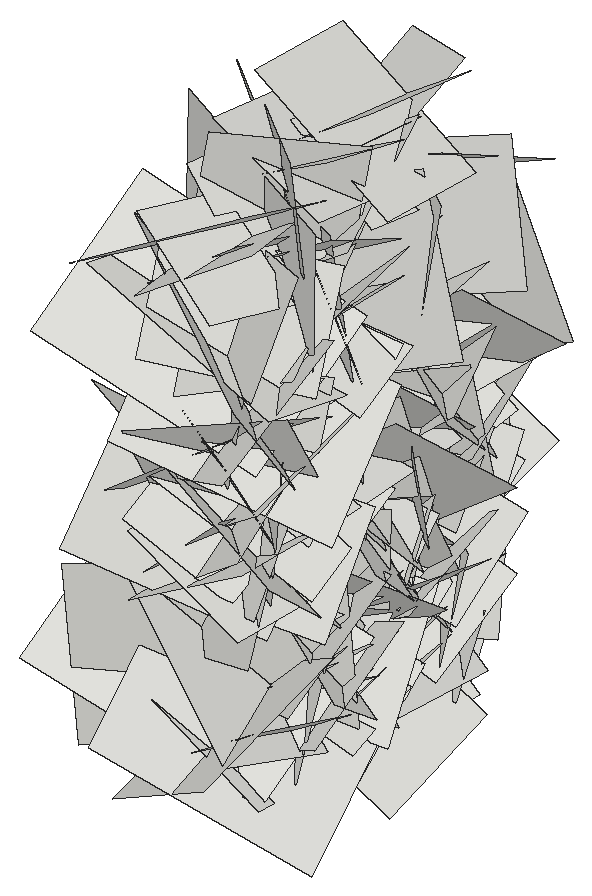
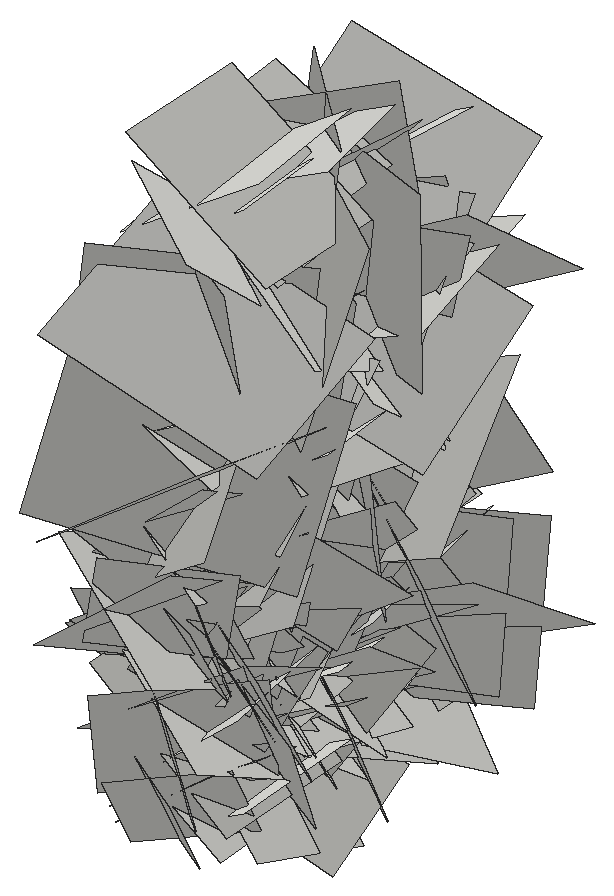
# SketchUp Ruby script. Lengths in inches.
U = 1.inch
M = Sketchup.active_model
def pt(a) = Geom::Point3d.new(a.map { |v| v * U })
def face(e, loops, mat)
  f = e.add_face(loops[0].map { |a| pt(a) })
  loops[1..].each { |l| e.add_face(l.map { |a| pt(a) }).erase! }
  f.material = f.back_material = mat if mat
  f
end
# faces: each face lists its corners as indices into pts; further lists are holes
def faces(e, pts, list, mat = nil) = list.each { |f| face(e, (f[0].is_a?(Array) ? f : [f]).map { |l| l.map { |i| pts[i] } }, mat) }
# xy, xz, yz: faces in a plane at the given z, y or x. An outline is a flat list of corners, or four numbers for a rectangle; further outlines are holes
def ring(l) = l.size == 4 ? [[l[0], l[1]], [l[2], l[1]], [l[2], l[3]], [l[0], l[3]]] : l.each_slice(2).to_a
def flat(e, list, mat, &to3) = list.each { |f| face(e, (f[0].is_a?(Array) ? f : [f]).map { |l| ring(l).map { |u, v| to3.(u, v) } }, mat) }
def xy(e, z, list, mat = nil) = flat(e, list, mat) { |x, y| [x, y, z] }
def xz(e, y, list, mat = nil) = flat(e, list, mat) { |x, z| [x, y, z] }
def yz(e, x, list, mat = nil) = flat(e, list, mat) { |y, z| [x, y, z] }
def lines(e, pts, list) = list.each { |a, b| e.add_line(pt(pts[a]), pt(pts[b])) }
# prism: a flat outline (further loops are holes) pulled along v
def prism(e, loops, v, mat = nil)
  f = face(e, loops, mat); d = Geom::Vector3d.new(v.map { |x| x * U })
  f.pushpull(f.normal.samedirection?(d) ? d.length : -d.length)
end
def box(e, o, s, mat = nil) = prism(e, [[o, [o[0] + s[0], o[1], o[2]], [o[0] + s[0], o[1] + s[1], o[2]], [o[0], o[1] + s[1], o[2]]]], [0, 0, s[2]], mat)
def at(x, y, z, deg = 0) = Geom::Transformation.translation(pt([x, y, z])) * Geom::Transformation.rotation(ORIGIN, Z_AXIS, deg.degrees)
def axes(o, x, y, z) = Geom::Transformation.new([*x, 0, *y, 0, *z, 0, *pt(o).to_a, 1])
def part(name) = M.definitions.add(name)
# library, detail: a bought-in or finely detailed component or shape, given as its bounding box
def library(name, o, s) = part(name).tap { |d| box(d.entities, o, s) }
def detail(e, o, s) = box(e.add_group.entities, o, s)
def put(e, d, t, mat = nil) = e.add_instance(d, t).tap { |i| i.material = mat if mat }
def group(e, t, mat = nil) = e.add_group.tap { |g| g.transformation = t; g.material = mat if mat }.entities
root = M.entities
c1 = part("Component\#6")
p = [[0.01,0,0],[0,3.24,4.54],[4.32,3.24,4.54],[4.33,0,0]]
faces(c1.entities,p,[[0,1,2,3]])
put(root,c1,axes([18.5,141,38.04],[-0.14868,1.2474,-0.57055],[-0.09146,-0.58042,-1.24775],[-1.45112,-0.09122,0.1371]))
put(root,c1,axes([18.5,143.09,24.72],[-0.05768,-1.1082,-0.74759],[-0.23067,-0.73089,1.09928],[-1.3981,0.16631,-0.15052]))
put(root,c1,axes([18.5,137.42,26.21],[-0.14568,0.69276,1.17725],[-0.03045,1.18146,-0.69859],[-1.44759,-0.09457,-0.10377]))
put(root,c1,axes([18.5,142.63,35.02],[-0.11092,-0.98462,-0.77371],[-0.1183,-0.76598,0.98988],[-1.32209,0.15114,-0.02366]))
put(root,c1,axes([18.5,142.42,32.89],[-0.18672,-0.42722,1.28431],[0.1337,1.28432,0.44452],[-1.42847,0.17605,-0.12627]))
put(root,c1,axes([18.5,139.39,34.34],[-0.15089,0.92592,0.71699],[-0.08883,0.71236,-0.93659],[-1.23815,-0.16395,-0.02018]))
put(root,c1,axes([18.5,140.25,33.3],[0.10371,-0.10781,1.29757],[-0.22808,1.282,0.12274],[-1.36119,-0.22303,0.07829]))
put(root,c1,axes([18.5,145.83,38.68],[0.04371,1.09164,-0.51046],[-0.28885,-0.48908,-1.06793],[-1.24431,0.15188,0.22998]))
put(root,c1,axes([18.5,141.15,27.9],[-0.10356,0.25866,-1.08582],[-0.18317,-1.08033,-0.24181],[-1.16891,0.14638,0.13409]))
put(root,c1,axes([18.5,141.71,25.57],[0.24627,-1.07768,0.84944],[-0.21085,0.82598,1.10232],[-1.43917,-0.30542,-0.01615]))
put(root,c1,axes([18.5,141.72,37.36],[-0.19445,0.97106,0.50245],[0.00165,0.50971,-0.98451],[-1.15895,-0.1622,-0.0857]))
put(root,c1,axes([18.5,149.48,27.53],[-0.05839,-0.93868,-0.8352],[0.07486,-0.83699,0.93604],[-1.32974,-0.0059,0.08937]))
put(root,c1,axes([18.5,145.76,27.48],[-0.11303,-0.66031,-0.96553],[0.02355,-0.9705,0.66125],[-1.23968,0.04176,0.1006]))
put(root,c1,axes([18.5,141.59,27.99],[0.06396,0.08339,-1.32201],[0.02487,-1.32324,-0.0824],[-1.4039,-0.01964,-0.06169]))
put(root,c1,axes([18.5,150.86,30.47],[-0.14962,-1.13409,-0.09371],[0.03493,-0.09847,1.14197],[-1.20573,0.13788,0.04471]))
put(root,c1,axes([18.5,144,25.2],[-0.04504,0.58566,0.95802],[-0.11757,0.95183,-0.5868],[-1.18441,-0.11675,0.02182]))
put(root,c1,axes([18.5,143.97,23.32],[-0.18437,0.48358,0.83906],[-0.16998,0.82633,-0.50949],[-1.01237,-0.22682,-0.06726]))
put(root,c1,axes([18.5,142.6875,32.73],[0.11413,-1.14483,0.29443],[-0.2702,0.26621,1.12831],[-1.22353,-0.16558,-0.2217]))
put(root,c1,axes([18.5,143.42,27.33],[-0.08667,-0.86973,1.01008],[0.23887,0.9884,0.86929],[-1.39256,0.22367,0.08625]))
put(root,c1,axes([18.5,141.2,30.22],[-0.14348,-0.5033,-0.91823],[-0.06175,-0.92081,0.51331],[-1.10823,0.11647,0.09028]))
put(root,c1,axes([18.5,141.99,33.2],[-0.15631,-0.03731,1.01998],[-0.08418,1.02787,0.02612],[-1.07863,-0.07482,-0.14985]))
put(root,c1,axes([18.5,146.73,29.36],[0.09029,-1.26195,0.03468],[-0.03892,0.03227,1.26436],[-1.33761,-0.08612,-0.03444]))
put(root,c1,axes([18.5,149.09,36.34],[0.1737,0.35213,-1.24285],[-0.08,-1.24806,-0.36356],[-1.36694,0.11779,-0.13666]))
put(root,c1,axes([18.5,137.65,40.3125],[-0.15365,0.92766,-0.3555],[-0.07441,-0.36793,-0.93147],[-1.05042,-0.10963,0.11798]))
put(root,c1,axes([18.5,140.69,35.43],[-0.02714,1.22478,0.26938],[0.1382,0.27058,-1.21783],[-1.3221,0.00314,-0.13283]))
put(root,c1,axes([18.5,138.43,27.8],[-0.10648,0.28124,1.16655],[0.16097,1.1642,-0.2676],[-1.26174,0.12479,-0.13259]))
put(root,c1,axes([14.53,147.9,27.03],[-0.12769,0.03013,0.63893],[-0.01482,0.64988,-0.03329],[0.67785,0.01989,0.11963]))
put(root,c1,axes([18.5,139.67,30.68],[0.09112,-0.77438,0.96294],[0.03313,0.96632,0.77431],[-1.3094,-0.02944,0.0866]))
put(root,c1,axes([14.53,144.97,35.07],[-0.07722,-0.5315,-0.34657],[-0.05738,-0.34237,0.53643],[0.67013,-0.09056,0.006]))
put(root,c1,axes([14.53,140.39,26.94],[-0.03872,-0.62994,0.14227],[-0.11345,0.14643,0.62088],[0.67508,-0.01152,0.1125]))
put(root,c1,axes([14.53,149.56,39.6],[-0.17317,-0.50739,-0.45031],[0.03865,-0.46908,0.51531],[0.71806,-0.09712,-0.13634]))
put(root,c1,axes([14.53,141.05,35.76],[-0.06877,-0.60814,0.14272],[-0.00885,0.14432,0.61116],[0.66208,-0.06124,0.02299]))
put(root,c1,axes([18.5,145.04,25.97],[0.0145,-0.85349,0.83598],[0.13626,0.83223,0.84756],[-1.25903,0.08024,0.10136]))
put(root,c1,axes([14.53,149.12,29.1],[-0.10824,-0.19319,-0.65872],[-0.02698,-0.66445,0.19881],[0.72715,-0.05341,-0.09068]))
put(root,c1,axes([18.5,139.49,21.74],[-0.04906,0.46783,0.90513],[-0.0041,0.90598,-0.46846],[-1.08001,-0.02469,-0.03934]))
put(root,c1,axes([14.53,142.28,27.34],[-0.09885,-0.42767,0.49172],[0.03253,0.4933,0.43487],[0.69002,-0.08452,0.04994]))
put(root,c1,axes([14.53,142.8,24.59],[-0.06246,-0.31977,0.5346],[0.03506,0.53462,0.32343],[0.65938,-0.05871,0.03344]))
put(root,c1,axes([18.5,138.75,33.42],[-0.07987,0.93748,-0.3836],[0.04246,-0.3816,-0.94046],[-1.07286,-0.0849,-0.00867]))
put(root,c1,axes([14.53,145.49,24.46],[-0.14807,-0.32942,-0.64401],[0.00647,-0.65643,0.33444],[0.76675,-0.05808,-0.12719]))
put(root,c1,axes([18.5,141.41,21.99],[-0.04242,-1.10503,0.33762],[0.18816,0.32793,1.09436],[-1.21025,0.08972,0.15831]))
put(root,c1,axes([18.5,142.58,23.75],[-0.11698,0.88265,-0.34817],[0.00423,-0.35009,-0.88876],[-1.00576,-0.10414,0.03675]))
put(root,c1,axes([18.5,145.05,38.54],[0.26561,0.06521,-1.32838],[0.06869,-1.35074,-0.05408],[-1.4081,-0.05359,-0.25321]))
put(root,c1,axes([18.5,146.5,19.86],[-0.14062,-0.87102,0.18651],[-0.03259,0.19294,0.87915],[-0.94365,0.12313,-0.05815]))
put(root,c1,axes([18.5,143.41,32.67],[0.00295,0.89075,-0.72818],[0.15415,-0.72261,-0.88339],[-1.20976,-0.08991,-0.11434]))
put(root,c1,axes([14.53,139.71,39.61],[0.08624,0.67106,-0.00672],[-0.16105,0.01183,-0.6586],[0.69289,-0.08077,-0.15225]))
put(root,c1,axes([18.5,144.65,25.96],[-0.15377,0.53431,0.65108],[-0.06081,0.65286,-0.54856],[-0.89071,-0.13681,-0.07495]))
put(root,c1,axes([14.53,144.73,33.27],[-0.16555,-0.76551,-0.15352],[0.02389,-0.16091,0.77946],[0.82725,-0.14855,-0.05323]))
put(root,c1,axes([14.53,146.45,21.25],[-0.00375,0.2874,0.54008],[0.0654,0.5375,-0.28562],[0.64519,-0.05282,0.03209]))
put(root,c1,axes([14.53,136.92,29.78],[0.03864,0.57092,0.32429],[-0.05823,0.3263,-0.56829],[0.69355,-0.00442,-0.06578]))
put(root,c1,axes([14.53,144.18,33.46],[-0.08879,-0.56105,-0.39599],[0.0694,-0.40364,0.55803],[0.72461,-0.03009,-0.10197]))
put(root,c1,axes([18.5,149.17,29.19],[-0.22051,-0.77582,-0.34275],[0.07369,-0.36732,0.78924],[-0.89602,0.16072,0.14925]))
put(root,c1,axes([14.53,141.16,33.73],[0.01034,-0.20439,-0.70125],[-0.11317,-0.69418,0.20085],[0.76594,-0.09981,0.03914]))
put(root,c1,axes([14.53,145.72,37.21],[0.0202,-0.65006,0.07365],[-0.02062,0.07308,0.65011],[0.69316,0.02112,0.01719]))
put(root,c1,axes([14.53,146.3,23.53],[-0.0913,-0.50535,0.50896],[0.05568,0.5068,0.51209],[0.75823,-0.09807,0.02368]))
put(root,c1,axes([14.53,145.7,22.51],[-0.08358,0.19729,0.79599],[-0.0899,0.79341,-0.20506],[0.86462,0.10156,0.05562]))
put(root,c1,axes([18.5,145.12,23.07],[0.0526,-0.82286,-0.58821],[-0.0059,-0.58914,0.82367],[-1.07215,-0.03713,-0.03339]))
put(root,c1,axes([18.5,137.68,27.62],[-0.00267,0.49736,0.77514],[-0.05686,0.77375,-0.49665],[-0.97459,-0.04651,0.02685]))
put(root,c1,axes([18.5,136.3,32.46],[0.17238,0.91042,0.71253],[0.07022,0.71102,-0.92361],[-1.22345,0.16908,0.04738]))
put(root,c1,axes([14.53,137.77,24.11],[-0.1419,0.78136,-0.16109],[0.04598,-0.15597,-0.79258],[0.84441,0.13979,0.01609]))
put(root,c1,axes([14.53,143.53,22.21],[-0.15224,-0.84766,-0.36991],[-0.10957,-0.35729,0.85887],[0.97421,-0.17265,0.03879]))
put(root,c1,axes([18.5,135.48,23.28],[0.21581,1.04519,0.5846],[0.09636,0.57779,-1.06467],[-1.26577,0.22219,0.01862]))
put(root,c1,axes([14.53,145.6,27.28],[0.00806,0.29423,-0.56577],[0.12293,-0.55701,-0.28812],[0.6647,0.09945,0.06014]))
put(root,c1,axes([18.5,141.63,23.18],[0.01995,1.00092,0.30572],[0.13829,0.30114,-0.99396],[-1.10071,0.05598,-0.11933]))
put(root,c1,axes([18.5,145.42,24.52],[0.2647,-0.88765,0.75819],[0.01358,0.77738,0.90589],[-1.23735,-0.18136,0.17214]))
put(root,c1,axes([14.53,144.6,22.65],[-0.17478,-0.82558,-0.09028],[0.09417,-0.10904,0.83495],[0.87528,-0.15312,-0.10786]))
put(root,c1,axes([18.5,142.67,41.25],[0.05619,0.9574,-0.08237],[-0.00834,-0.08206,-0.95886],[-1.01856,0.05349,0.00331]))
put(root,c1,axes([18.5,148.52,32.35],[-0.08011,-0.79067,-0.06214],[-0.07476,-0.05548,0.79163],[-0.83736,0.0806,-0.06473]))
put(root,c1,axes([14.53,140.84,40.56],[-0.05261,0.712,-0.12967],[0.10362,-0.12219,-0.70833],[0.7601,0.06594,0.08758]))
put(root,c1,axes([14.53,143.38,25.93],[-0.00088,-0.66729,0.07011],[0.1194,0.06898,0.65784],[0.70113,-0.01259,-0.11194]))
put(root,c1,axes([14.53,144.05,31.85],[-0.11078,0.17753,-0.74918],[0.12323,-0.74375,-0.19246],[0.80677,0.13798,-0.07348]))
put(root,c1,axes([18.5,138.53,29.67],[-0.03677,-0.4198,0.69058],[-0.10131,0.68849,0.41374],[-0.85065,-0.06385,-0.07912]))
put(root,c1,axes([18.5,150.98,27.43],[-0.11329,-0.77541,-0.3635],[0.07754,-0.37325,0.77469],[-0.90445,0.06513,0.11195]))
put(root,c1,axes([18.5,149.13,24.11],[0.03147,-0.85153,-0.39996],[0.02133,-0.3995,0.85202],[-0.997,-0.03542,0.00561]))
put(root,c1,axes([18.5,144.71,33.13],[0.16995,0.04512,1.05289],[0.00982,1.0649,-0.04705],[-1.11704,0.01623,0.15977]))
put(root,c1,axes([14.53,143.64,28.51],[0.01569,-0.00258,-0.72773],[0.02057,-0.72762,0.00297],[0.77112,0.01947,0.01473]))
put(root,c1,axes([18.5,137.85,30.84],[0.06669,0.91948,0.38333],[0.06841,0.37952,-0.92095],[-1.05374,0.08283,-0.03553]))
put(root,c1,axes([18.5,147.08,31.53],[0.0186,0.21399,-0.90436],[0.04027,-0.90393,-0.21315],[-0.98427,-0.03294,-0.02581]))
put(root,c1,axes([14.53,144.98,23.12],[0.11015,0.70988,0.06167],[-0.04855,0.06885,-0.71532],[0.75374,-0.09931,-0.05509]))
put(root,c1,axes([14.53,140.76,35.5625],[0.0095,0.80566,-0.00603],[-0.04784,-0.00552,-0.80445],[0.85268,-0.00929,-0.04507]))
put(root,c1,axes([14.53,146.7,34.04],[-0.22474,0.77203,-0.6543],[-0.03576,-0.67353,-0.78378],[1.07212,0.13937,-0.1633]))
put(root,c1,axes([18.5,141.61,27.46],[0.15544,0.8369,-0.58263],[0.03072,-0.5918,-0.84279],[-1.08048,0.10358,-0.10778]))
put(root,c1,axes([18.5,145.6875,25.3],[0.21495,-0.77208,-0.77151],[0.06755,-0.77499,0.79232],[-1.15499,-0.18901,-0.09724]))
put(root,c1,axes([18.5,147.86,21.63],[0.08807,-1.00346,0.13322],[0.11481,0.14172,0.99989],[-1.06685,-0.06759,0.1186]))
put(root,c1,axes([14.53,139.84,37.375],[0.13047,0.02824,0.77],[-0.11824,0.77221,-0.01049],[0.80815,0.10842,-0.12584]))
put(root,c1,axes([18.5,144.76,23.61],[-0.10873,-0.7568,0.02149],[0.01122,0.02025,0.76368],[-0.80245,0.10283,0.00777]))
put(root,c1,axes([14.53,149.44,28.46],[-0.01637,-0.35652,-0.61871],[0.18604,-0.60176,0.34238],[0.7337,0.14463,-0.10062]))
put(root,c1,axes([14.53,137.14,29.31],[0.00249,0.75761,-0.01469],[0.08098,-0.01485,-0.75375],[0.79913,-0.00085,0.07643]))
put(root,c1,axes([14.53,137.53,34.5],[-0.08019,0.3809,0.76753],[0.04804,0.77121,-0.37826],[0.90698,-0.00717,0.08789]))
put(root,c1,axes([18.5,139.47,36.72],[-0.15825,-0.66033,0.08813],[-0.02764,0.09604,0.67542],[-0.70562,0.14433,-0.04622]))
put(root,c1,axes([14.53,139.47,36.72],[0.15825,-0.66033,0.08813],[0.02764,0.09604,0.67542],[0.70562,0.14433,-0.04622]))
put(root,c1,axes([18.5,137.53,34.5],[0.08019,0.3809,0.76753],[-0.04804,0.77121,-0.37826],[-0.90698,-0.00717,0.08789]))
put(root,c1,axes([18.5,137.14,29.31],[-0.00249,0.75761,-0.01469],[-0.08098,-0.01485,-0.75375],[-0.79913,-0.00085,0.07643]))
put(root,c1,axes([18.5,149.44,28.46],[0.01637,-0.35652,-0.61871],[-0.18604,-0.60176,0.34238],[-0.7337,0.14463,-0.10062]))
put(root,c1,axes([14.53,144.76,23.61],[0.10873,-0.7568,0.02149],[-0.01122,0.02025,0.76368],[0.80245,0.10283,0.00777]))
put(root,c1,axes([18.5,139.84,37.375],[-0.13047,0.02824,0.77],[0.11824,0.77221,-0.01049],[-0.80815,0.10842,-0.12584]))
put(root,c1,axes([14.53,147.86,21.63],[-0.08807,-1.00346,0.13322],[-0.11481,0.14172,0.99989],[1.06685,-0.06759,0.1186]))
put(root,c1,axes([14.53,145.6875,25.3],[-0.21495,-0.77208,-0.77151],[-0.06755,-0.77499,0.79232],[1.15499,-0.18901,-0.09724]))
put(root,c1,axes([14.53,141.61,27.46],[-0.15544,0.8369,-0.58263],[-0.03072,-0.5918,-0.84279],[1.08048,0.10358,-0.10778]))
put(root,c1,axes([18.5,146.7,34.04],[0.22474,0.77203,-0.6543],[0.03576,-0.67353,-0.78378],[-1.07212,0.13937,-0.1633]))
put(root,c1,axes([18.5,140.76,35.5625],[-0.0095,0.80566,-0.00603],[0.04784,-0.00552,-0.80445],[-0.85268,-0.00929,-0.04507]))
put(root,c1,axes([18.5,144.98,23.12],[-0.11015,0.70988,0.06167],[0.04855,0.06885,-0.71532],[-0.75374,-0.09931,-0.05509]))
put(root,c1,axes([14.53,147.08,31.53],[-0.0186,0.21399,-0.90436],[-0.04027,-0.90393,-0.21315],[0.98427,-0.03294,-0.02581]))
put(root,c1,axes([14.53,137.85,30.84],[-0.06669,0.91948,0.38333],[-0.06841,0.37952,-0.92095],[1.05374,0.08283,-0.03553]))
put(root,c1,axes([18.5,143.64,28.51],[-0.01569,-0.00258,-0.72773],[-0.02057,-0.72762,0.00297],[-0.77112,0.01947,0.01473]))
put(root,c1,axes([14.53,144.71,33.13],[-0.16995,0.04512,1.05289],[-0.00982,1.0649,-0.04705],[1.11704,0.01623,0.15977]))
put(root,c1,axes([14.53,149.13,24.11],[-0.03147,-0.85153,-0.39996],[-0.02133,-0.3995,0.85202],[0.997,-0.03542,0.00561]))
put(root,c1,axes([14.53,150.98,27.43],[0.11329,-0.77541,-0.3635],[-0.07754,-0.37325,0.77469],[0.90445,0.06513,0.11195]))
put(root,c1,axes([14.53,138.53,29.67],[0.03677,-0.4198,0.69058],[0.10131,0.68849,0.41374],[0.85065,-0.06385,-0.07912]))
put(root,c1,axes([18.5,144.05,31.85],[0.11078,0.17753,-0.74918],[-0.12323,-0.74375,-0.19246],[-0.80677,0.13798,-0.07348]))
put(root,c1,axes([18.5,143.38,25.93],[0.00088,-0.66729,0.07011],[-0.1194,0.06898,0.65784],[-0.70113,-0.01259,-0.11194]))
put(root,c1,axes([18.5,140.84,40.56],[0.05261,0.712,-0.12967],[-0.10362,-0.12219,-0.70833],[-0.7601,0.06594,0.08758]))
put(root,c1,axes([14.53,148.52,32.35],[0.08011,-0.79067,-0.06214],[0.07476,-0.05548,0.79163],[0.83736,0.0806,-0.06473]))
put(root,c1,axes([14.53,142.67,41.25],[-0.05619,0.9574,-0.08237],[0.00834,-0.08206,-0.95886],[1.01856,0.05349,0.00331]))
put(root,c1,axes([18.5,144.6,22.65],[0.17478,-0.82558,-0.09028],[-0.09417,-0.10904,0.83495],[-0.87528,-0.15312,-0.10786]))
put(root,c1,axes([14.53,145.42,24.52],[-0.2647,-0.88765,0.75819],[-0.01358,0.77738,0.90589],[1.23735,-0.18136,0.17214]))
put(root,c1,axes([14.53,141.63,23.18],[-0.01995,1.00092,0.30572],[-0.13829,0.30114,-0.99396],[1.10071,0.05598,-0.11933]))
put(root,c1,axes([18.5,145.6,27.28],[-0.00806,0.29423,-0.56577],[-0.12293,-0.55701,-0.28812],[-0.6647,0.09945,0.06014]))
put(root,c1,axes([14.53,135.48,23.28],[-0.21581,1.04519,0.5846],[-0.09636,0.57779,-1.06467],[1.26577,0.22219,0.01862]))
put(root,c1,axes([18.5,143.53,22.21],[0.15224,-0.84766,-0.36991],[0.10957,-0.35729,0.85887],[-0.97421,-0.17265,0.03879]))
put(root,c1,axes([18.5,137.77,24.11],[0.1419,0.78136,-0.16109],[-0.04598,-0.15597,-0.79258],[-0.84441,0.13979,0.01609]))
put(root,c1,axes([14.53,136.3,32.46],[-0.17238,0.91042,0.71253],[-0.07022,0.71102,-0.92361],[1.22345,0.16908,0.04738]))
put(root,c1,axes([14.53,137.68,27.62],[0.00267,0.49736,0.77514],[0.05686,0.77375,-0.49665],[0.97459,-0.04651,0.02685]))
put(root,c1,axes([14.53,145.12,23.07],[-0.0526,-0.82286,-0.58821],[0.0059,-0.58914,0.82367],[1.07215,-0.03713,-0.03339]))
put(root,c1,axes([18.5,145.7,22.51],[0.08358,0.19729,0.79599],[0.0899,0.79341,-0.20506],[-0.86462,0.10156,0.05562]))
put(root,c1,axes([18.5,146.3,23.53],[0.0913,-0.50535,0.50896],[-0.05568,0.5068,0.51209],[-0.75823,-0.09807,0.02368]))
put(root,c1,axes([18.5,145.72,37.21],[-0.0202,-0.65006,0.07365],[0.02062,0.07308,0.65011],[-0.69316,0.02112,0.01719]))
put(root,c1,axes([18.5,141.16,33.73],[-0.01034,-0.20439,-0.70125],[0.11317,-0.69418,0.20085],[-0.76594,-0.09981,0.03914]))
put(root,c1,axes([14.53,149.17,29.19],[0.22051,-0.77582,-0.34275],[-0.07369,-0.36732,0.78924],[0.89602,0.16072,0.14925]))
put(root,c1,axes([18.5,144.18,33.46],[0.08879,-0.56105,-0.39599],[-0.0694,-0.40364,0.55803],[-0.72461,-0.03009,-0.10197]))
put(root,c1,axes([18.5,136.92,29.78],[-0.03864,0.57092,0.32429],[0.05823,0.3263,-0.56829],[-0.69355,-0.00442,-0.06578]))
put(root,c1,axes([18.5,146.45,21.25],[0.00375,0.2874,0.54008],[-0.0654,0.5375,-0.28562],[-0.64519,-0.05282,0.03209]))
put(root,c1,axes([18.5,144.73,33.27],[0.16555,-0.76551,-0.15352],[-0.02389,-0.16091,0.77946],[-0.82725,-0.14855,-0.05323]))
put(root,c1,axes([14.53,144.65,25.96],[0.15377,0.53431,0.65108],[0.06081,0.65286,-0.54856],[0.89071,-0.13681,-0.07495]))
